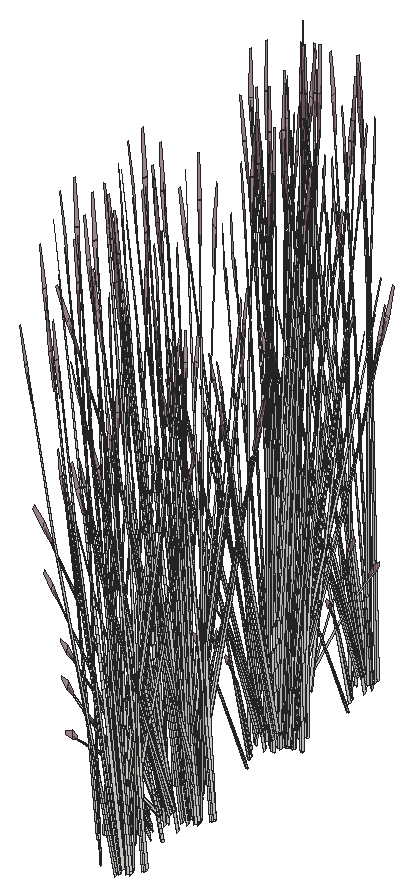
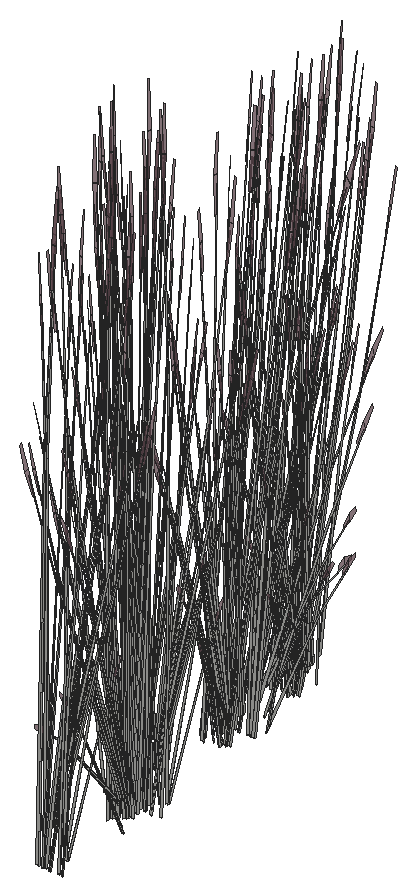
# SketchUp Ruby script. Lengths in inches.
U = 1.inch
M = Sketchup.active_model
def pt(a) = Geom::Point3d.new(a.map { |v| v * U })
def face(e, loops, mat)
  f = e.add_face(loops[0].map { |a| pt(a) })
  loops[1..].each { |l| e.add_face(l.map { |a| pt(a) }).erase! }
  f.material = f.back_material = mat if mat
  f
end
# faces: each face lists its corners as indices into pts; further lists are holes
def faces(e, pts, list, mat = nil) = list.each { |f| face(e, (f[0].is_a?(Array) ? f : [f]).map { |l| l.map { |i| pts[i] } }, mat) }
# xy, xz, yz: faces in a plane at the given z, y or x. An outline is a flat list of corners, or four numbers for a rectangle; further outlines are holes
def ring(l) = l.size == 4 ? [[l[0], l[1]], [l[2], l[1]], [l[2], l[3]], [l[0], l[3]]] : l.each_slice(2).to_a
def flat(e, list, mat, &to3) = list.each { |f| face(e, (f[0].is_a?(Array) ? f : [f]).map { |l| ring(l).map { |u, v| to3.(u, v) } }, mat) }
def xy(e, z, list, mat = nil) = flat(e, list, mat) { |x, y| [x, y, z] }
def xz(e, y, list, mat = nil) = flat(e, list, mat) { |x, z| [x, y, z] }
def yz(e, x, list, mat = nil) = flat(e, list, mat) { |y, z| [x, y, z] }
def lines(e, pts, list) = list.each { |a, b| e.add_line(pt(pts[a]), pt(pts[b])) }
# prism: a flat outline (further loops are holes) pulled along v
def prism(e, loops, v, mat = nil)
  f = face(e, loops, mat); d = Geom::Vector3d.new(v.map { |x| x * U })
  f.pushpull(f.normal.samedirection?(d) ? d.length : -d.length)
end
def box(e, o, s, mat = nil) = prism(e, [[o, [o[0] + s[0], o[1], o[2]], [o[0] + s[0], o[1] + s[1], o[2]], [o[0], o[1] + s[1], o[2]]]], [0, 0, s[2]], mat)
def at(x, y, z, deg = 0) = Geom::Transformation.translation(pt([x, y, z])) * Geom::Transformation.rotation(ORIGIN, Z_AXIS, deg.degrees)
def axes(o, x, y, z) = Geom::Transformation.new([*x, 0, *y, 0, *z, 0, *pt(o).to_a, 1])
def part(name) = M.definitions.add(name)
# library, detail: a bought-in or finely detailed component or shape, given as its bounding box
def library(name, o, s) = part(name).tap { |d| box(d.entities, o, s) }
def detail(e, o, s) = box(e.add_group.entities, o, s)
def put(e, d, t, mat = nil) = e.add_instance(d, t).tap { |i| i.material = mat if mat }
def group(e, t, mat = nil) = e.add_group.tap { |g| g.transformation = t; g.material = mat if mat }.entities
root = M.entities
M.materials.add("LightPink_Translucent").color = [144, 107, 117]
M.materials["LightPink_Translucent"].alpha = 0.75
c1 = part("blade")
p = [[2.15,0.21,22],[0,0.17,0],[0.09,0.45,0],[2.18,0.31,22],[2.29,0.31,22],[0.38,0.45,0],
  [2.48,0.24,33],[2.49,0.24,33],[2.48,0.22,33]]
faces(c1.entities,p,[[0,1,2,3],[4,5,2,3],[6,3,4,7],[8,0,3,6]])
c2 = part("seeds")
p = [[0.3,-0.1,1.38],[-0.01,-0.03,1.59],[-0.01,-0.03,0.03],[0.14,-0.07,-0.07],[0.29,-0.03,3],[0.15,0.01,3.11]]
faces(c2.entities,p,[[0,1,2,3],[1,0,4,5]],"LightPink_Translucent")
c3 = part("blade with seeds")
put(c3.entities,c1,at(0,0,0))
put(c3.entities,c2,axes([2.4,0.25,30.99],[1.5799,-0.05474,1.17369],[-0.12525,1.92788,0.29478],[-0.07173,-0.02425,1.56792]))
put(root,c3,axes([405.85,331.17,-9.69],[0,0.54355,0.46235],[-0.57217,0,0],[0,-0.1238,1.46668]))
put(root,c3,axes([407.2,331.61,-9.94],[-0.30722,-0.45622,-0.41661],[0.46535,-0.32126,0.2005],[-0.09942,-0.05645,1.33761]))
put(root,c3,axes([406.93,331.78,-10.08],[-0.53199,-0.08911,-0.58063],[0.11226,-0.54969,-0.15239],[-0.15876,-0.06661,1.28164]))
put(root,c3,axes([406.36,332.62,-10.11],[-0.12013,-0.47362,-0.28847],[0.47712,-0.13449,0.28847],[-0.09619,-0.05462,1.29413]))
put(root,c3,axes([406.23,332.82,-10.12],[-0.47863,-0.27177,-0.46235],[0.28609,-0.48733,0],[-0.10901,-0.0619,1.46668]))
put(root,c3,axes([407.53,331.86,-9.52],[-0.51635,0.36087,-0.27094],[-0.34336,-0.5099,-0.46562],[-0.1274,-0.05178,1.4872]))
put(root,c3,axes([407.48,332.02,-9.5625],[-0.09866,0.48509,0.13483],[-0.48202,-0.0842,-0.38503],[-0.08772,-0.04981,1.18024]))
put(root,c3,axes([405.61,330.76,-7.3],[0.42502,0.15163,0.32977],[-0.12396,0.44238,-0.42575],[-0.17112,0.04056,0.81462]))
put(root,c3,axes([408.11,332.03,-9.7],[-0.49938,-0.43748,-0.23459],[0.42021,-0.49126,0.51337],[-0.13447,0.05118,1.56642]))
put(root,c3,axes([406.8,332.87,-9.69],[0.47863,0.27177,0.46235],[-0.28609,0.48733,0],[-0.10901,-0.0619,1.46668]))
put(root,c3,axes([406.52,333.15,-9.79],[-0.31974,0.54466,0],[-0.53494,-0.30375,-0.48057],[-0.12184,-0.06918,1.52448]))
put(root,c3,axes([407.86,331.93,-9.94],[-0.55535,0.03355,-0.41661],[-0.05022,-0.55698,0.2005],[-0.09942,0.05645,1.33761]))
put(root,c3,axes([405.78,337.88,-8.39],[0.1169,0.17452,1.59586],[-0.54019,0.14692,0.12904],[-0.12209,-0.27397,0.68222]))
put(root,c3,axes([408.47,333.23,-9.96],[-0.31576,-0.54657,-0.04789],[0.53494,-0.30375,0.48057],[-0.13182,0.05204,1.52373]))
put(root,c3,axes([406.67,336.73,-7.61],[-0.07822,-0.07621,1.62908],[-0.52201,0.04832,-0.25764],[-0.08331,-0.18228,0.13065]))
put(root,c3,axes([407.21,338.01,-7.36],[-0.24409,-0.44196,-0.66157],[0.50245,-0.2463,0.07984],[-0.05708,-0.21354,0.93586]))
put(root,c3,axes([405.63,337.42,-9.59],[-0.03097,0.17781,1.33163],[-0.45273,0.14885,-0.28638],[-0.10583,-0.22982,0.56934]))
put(root,c3,axes([408.33,333.16,-10.11],[-0.47712,-0.13449,-0.28847],[0.12013,-0.47362,0.28847],[-0.09619,0.05462,1.29413]))
put(root,c3,axes([405.68,331.82,-7.3],[0.44516,-0.07768,0.32977],[0.11755,0.44407,-0.42575],[-0.12757,0.11927,0.81462]))
put(root,c3,axes([407.03,337.93,-7.64],[-0.50273,-0.13626,-0.47583],[0.17232,-0.46717,-0.36857],[-0.0461,-0.18809,0.91046]))
put(root,c3,axes([406.13,336.48,-7.62],[-0.00954,0.06515,1.65179],[-0.47055,0.23645,-0.15608],[-0.13847,-0.12087,0.29231]))
put(root,c3,axes([404.67,333.08,-6.74],[0.45129,0.14509,-0.06041],[-0.13882,0.44656,-0.27392],[-0.07381,0.0678,0.90349]))
put(root,c3,axes([407.87,332.26,-10.08],[-0.34446,0.40855,-0.58063],[-0.42791,-0.37046,-0.15239],[-0.13803,0.10191,1.28164]))
put(root,c3,axes([406.03,337.63,-7.26],[0.56969,-0.13971,0.50064],[0.09887,0.54803,0.4128],[-0.13398,-0.16152,1.03595]))
put(root,c3,axes([407.46,337.9,-7.3125],[-0.50045,0.25306,-0.11324],[-0.24593,-0.44915,-0.62851],[-0.06603,-0.18927,0.95501]))
put(root,c3,axes([408.44,333.37,-10.12],[-0.47863,0.27177,-0.46235],[-0.28609,-0.48733,0],[-0.10901,0.0619,1.46668]))
put(root,c3,axes([405.47,337.14,-9.42],[0.26677,0.18918,1.06958],[-0.38851,0.11372,0.78586],[-0.08313,-0.14539,0.23558]))
put(root,c3,axes([405.96,337.79,-7.78],[-0.07899,-0.43781,-0.32977],[0.45153,-0.11561,0.42575],[-0.12128,-0.12546,0.81462]))
put(root,c3,axes([405.45,331.78,-7.3125],[0.47307,0.29971,-0.11324],[-0.27254,0.43404,-0.62851],[-0.13365,0.15087,0.95501]))
put(root,c3,axes([405.6875,332.14,-7.64],[0.13138,0.49631,-0.47583],[-0.49754,0.08682,-0.36857],[-0.14258,0.13331,0.91046]))
put(root,c3,axes([406.16,337.75,-7.6],[0.23243,-0.34529,0.05988],[0.331,0.20103,0.47138],[-0.10701,-0.1107,0.71878]))
put(root,c3,axes([405.26,337.71,-10.61],[-0.04954,0.0716,1.6421],[-0.50062,0.15438,-0.25086],[-0.12094,-0.14044,0.2797]))
put(root,c3,axes([406.28,332.71,-7.3],[0.34603,-0.28618,0.32977],[0.32756,0.32677,-0.42575],[-0.04984,0.16603,0.81462]))
put(root,c3,axes([406.09,339.67,-10.05],[-0.21003,-0.55738,-0.65031],[0.60499,-0.20074,-0.17068],[-0.02321,-0.18874,1.43544]))
put(root,c3,axes([408.6,331.13,-9.35],[-0.01397,-0.51177,1.31553],[0.63227,0.13266,0.557],[-0.14954,0.28003,1.24175]))
put(root,c3,axes([405.97,332.97,-7.6],[-0.42027,-0.02533,0.05988],[0.01152,-0.38243,0.47138],[-0.04398,0.14649,0.71878]))
put(root,c3,axes([406.1,333,-7.59],[-0.36417,-0.37086,0.447],[0.38674,-0.31985,0.36857],[-0.06718,0.174,0.92496]))
put(root,c3,axes([406.71,337.42,-10.02],[-0.35341,0.31182,-0.03625],[-0.32382,-0.34152,-0.16435],[-0.0228,-0.09677,0.54209]))
put(root,c3,axes([405.99,332.0625,-8.39],[0.09522,-0.18683,1.59586],[0.39947,0.38663,0.12904],[-0.18021,0.24097,0.68222]))
put(root,c3,axes([407.16,341.11,-8.9],[0.44194,0.21918,1.40854],[-0.43295,0.47219,0.557],[-0.19393,-0.27986,1.18082]))
put(root,c3,axes([406.1,333.11,-7.78],[-0.34603,0.28618,-0.32977],[-0.32756,-0.32677,0.42575],[-0.04984,0.16603,0.81462]))
put(root,c3,axes([404.91,333.03,-7.61],[-0.01271,0.10756,1.62908],[0.36076,0.37419,-0.25764],[-0.09444,0.17695,0.13065]))
put(root,c3,axes([406.0625,332.79,-6.97],[0.56206,0.02693,-0.12569],[-0.01536,0.50991,-0.69765],[-0.03904,0.19638,1.06006]))
put(root,c3,axes([406.23,338.15,-7.3],[0.07899,0.43781,0.32977],[-0.45153,0.11561,-0.42575],[-0.12128,-0.12546,0.81462]))
put(root,c3,axes([404.85,339.6,-10.12],[0,-0.54355,-0.46235],[0.57217,0,0],[0,-0.1238,1.46668]))
put(root,c3,axes([406.32,334.23,-9.42],[-0.01324,-0.32319,1.06958],[0.33072,0.23052,0.78586],[-0.06504,0.15405,0.23558]))
put(root,c3,axes([406.45,332.98,-7.34],[0.3661,0.36521,-0.52818],[-0.38674,0.31985,-0.40911],[-0.0557,0.18556,1.01061]))
put(root,c3,axes([406.05,333.53,-9.37],[0.46459,-0.09625,0.0606],[0.10681,0.38778,-0.80367],[-0.02945,0.1963,0.72038]))
put(root,c3,axes([405.09,339.61,-10.11],[0.35699,-0.33913,-0.28847],[0.35699,0.33913,0.28847],[0,-0.10923,1.29413]))
put(root,c3,axes([404.95,337.98,-10.02],[-0.14753,0.44383,-0.03625],[-0.45406,-0.13653,-0.16435],[-0.06894,-0.07259,0.54209]))
put(root,c3,axes([406.34,340.23,-9.52],[-0.57594,-0.25935,-0.27094],[0.27732,-0.5474,-0.46562],[-0.0181,-0.1344,1.4872]))
put(root,c3,axes([404.71,340.01,-9.79],[-0.63949,0,0],[0,-0.60749,-0.48057],[0,-0.13836,1.52448]))
put(root,c3,axes([406.33,332.8125,-7.03],[-0.01331,0.50278,-0.73435],[-0.56035,-0.03377,0.08862],[-0.05914,0.213,1.03881]))
put(root,c3,axes([404.87,334.13,-7.62],[0.05802,-0.03282,1.65179],[0.47954,0.21828,-0.15608],[-0.01127,0.18175,0.29231]))
put(root,c3,axes([405.9375,333.9375,-9.59],[0.16138,-0.08575,1.33163],[0.39845,0.25854,-0.28638],[-0.1186,0.22371,0.56934]))
put(root,c3,axes([405.2,339.85,-9.83],[-0.47569,0.45698,0.2864],[-0.47598,-0.45217,-0.33981],[-0.01661,-0.12977,1.53541]))
put(root,c3,axes([406.49,340.8,-9.73],[0.13555,-0.64407,-0.21817],[0.64269,0.11227,0.47743],[-0.1123,-0.08895,1.45677]))
put(root,c3,axes([406.15,333.52,-8.87],[0.01124,-0.2806,1.43727],[0.50537,0.14821,0.19862],[-0.04379,0.29905,0.67868]))
put(root,c3,axes([405.09,340.1,-9.69],[0,0.54355,0.46235],[-0.57217,0,0],[0,-0.1238,1.46668]))
put(root,c3,axes([406.44,340.54,-9.94],[-0.30722,-0.45622,-0.41661],[0.46535,-0.32126,0.2005],[-0.09942,-0.05645,1.33761]))
put(root,c3,axes([406.4,340.375,-9.47],[-0.24813,0.48978,0.41661],[-0.51557,-0.23571,-0.2005],[0,-0.1129,1.33761]))
put(root,c3,axes([406.5625,340.49,-9.8],[0.64638,0.11452,0.42607],[-0.13155,0.64678,0.16719],[-0.09446,-0.06245,1.47927]))
put(root,c3,axes([405.6,341.55,-10.11],[-0.12013,-0.47362,-0.28847],[0.47712,-0.13449,0.28847],[-0.09619,-0.05462,1.29413]))
put(root,c3,axes([406.22,341.52,-9.7],[0.54955,-0.14427,0.16428],[0.1357,0.53689,0.32672],[-0.04901,-0.07823,1.49371]))
put(root,c3,axes([405.47,341.76,-10.12],[-0.47863,-0.27177,-0.46235],[0.28609,-0.48733,0],[-0.10901,-0.0619,1.46668]))
put(root,c3,axes([406.77,340.8,-9.52],[-0.51635,0.36087,-0.27094],[-0.34336,-0.5099,-0.46562],[-0.1274,-0.05178,1.4872]))
put(root,c3,axes([406.72,340.95,-9.5625],[-0.09866,0.48509,0.13483],[-0.48202,-0.0842,-0.38503],[-0.08772,-0.04981,1.18024]))
put(root,c3,axes([407.35,340.96,-9.7],[-0.49938,-0.43748,-0.23459],[0.42021,-0.49126,0.51337],[-0.13447,0.05118,1.56642]))
put(root,c3,axes([406.04,341.8,-9.69],[0.47863,0.27177,0.46235],[-0.28609,0.48733,0],[-0.10901,-0.0619,1.46668]))
put(root,c3,axes([405.76,342.08,-9.79],[-0.31974,0.54466,0],[-0.53494,-0.30375,-0.48057],[-0.12184,-0.06918,1.52448]))
put(root,c3,axes([407.1,340.87,-9.94],[-0.55535,0.03355,-0.41661],[-0.05022,-0.55698,0.2005],[-0.09942,0.05645,1.33761]))
put(root,c3,axes([407.71,342.16,-9.96],[-0.31576,-0.54657,-0.04789],[0.53494,-0.30375,0.48057],[-0.13182,0.05204,1.52373]))
put(root,c3,axes([407.57,342.09,-10.11],[-0.47712,-0.13449,-0.28847],[0.12013,-0.47362,0.28847],[-0.09619,0.05462,1.29413]))
put(root,c3,axes([404.92,340.76,-7.3],[0.44516,-0.07768,0.32977],[0.11755,0.44407,-0.42575],[-0.12757,0.11927,0.81462]))
put(root,c3,axes([407.49,340.72,-9.52],[0.05959,0.62022,-0.27094],[-0.62068,0.0375,-0.46562],[-0.1093,0.08261,1.4872]))
put(root,c3,axes([403.91,342.02,-6.74],[0.45129,0.14509,-0.06041],[-0.13882,0.44656,-0.27392],[-0.07381,0.0678,0.90349]))
put(root,c3,axes([407.11,341.19,-10.08],[-0.34446,0.40855,-0.58063],[-0.42791,-0.37046,-0.15239],[-0.13803,0.10191,1.28164]))
put(root,c3,axes([407.68,342.31,-10.12],[-0.47863,0.27177,-0.46235],[-0.28609,-0.48733,0],[-0.10901,0.0619,1.46668]))
put(root,c3,axes([404.69,340.72,-7.3125],[0.47307,0.29971,-0.11324],[-0.27254,0.43404,-0.62851],[-0.13365,0.15087,0.95501]))
put(root,c3,axes([405.52,341.64,-7.3],[0.34603,-0.28618,0.32977],[0.32756,0.32677,-0.42575],[-0.04984,0.16603,0.81462]))
put(root,c3,axes([407.84,340.06,-9.35],[-0.01397,-0.51177,1.31553],[0.63227,0.13266,0.557],[-0.14954,0.28003,1.24175]))
put(root,c3,axes([405.21,341.9,-7.6],[-0.42027,-0.02533,0.05988],[0.01152,-0.38243,0.47138],[-0.04398,0.14649,0.71878]))
put(root,c3,axes([405.34,341.9375,-7.59],[-0.36417,-0.37086,0.447],[0.38674,-0.31985,0.36857],[-0.06718,0.174,0.92496]))
put(root,c3,axes([405.34,342.05,-7.78],[-0.34603,0.28618,-0.32977],[-0.32756,-0.32677,0.42575],[-0.04984,0.16603,0.81462]))
put(root,c3,axes([405.3,341.72,-6.97],[0.56206,0.02693,-0.12569],[-0.01536,0.50991,-0.69765],[-0.03904,0.19638,1.06006]))
put(root,c3,axes([405.5625,343.16,-9.42],[-0.01324,-0.32319,1.06958],[0.33072,0.23052,0.78586],[-0.06504,0.15405,0.23558]))
put(root,c3,axes([405.6875,341.91,-7.34],[0.3661,0.36521,-0.52818],[-0.38674,0.31985,-0.40911],[-0.0557,0.18556,1.01061]))
put(root,c3,axes([405.29,342.46,-9.37],[0.46459,-0.09625,0.0606],[0.10681,0.38778,-0.80367],[-0.02945,0.1963,0.72038]))
put(root,c3,axes([405.57,341.74,-7.03],[-0.01331,0.50278,-0.73435],[-0.56035,-0.03377,0.08862],[-0.05914,0.213,1.03881]))
put(root,c3,axes([404.11,343.07,-7.62],[0.05802,-0.03282,1.65179],[0.47954,0.21828,-0.15608],[-0.01127,0.18175,0.29231]))
put(root,c3,axes([406.1,341.39,-8.39],[-0.01252,-0.20862,1.59586],[0.54251,0.1384,0.12904],[-0.03356,0.2973,0.68222]))
put(root,c3,axes([405.18,342.87,-9.59],[0.16138,-0.08575,1.33163],[0.39845,0.25854,-0.28638],[-0.1186,0.22371,0.56934]))
put(root,c3,axes([404.54,351.54,-7.36],[-0.24409,-0.44196,-0.66157],[0.50245,-0.2463,0.07984],[-0.05708,-0.21354,0.93586]))
put(root,c3,axes([404.12,350.5625,-10.61],[-0.08578,0.01958,1.6421],[-0.47437,-0.22044,-0.25086],[0.00796,-0.18387,0.2797]))
put(root,c3,axes([405.39,342.45,-8.87],[0.01124,-0.2806,1.43727],[0.50537,0.14821,0.19862],[-0.04379,0.29905,0.67868]))
put(root,c3,axes([404.58,351.17,-7.78],[0.15418,-0.41799,-0.32977],[0.44981,0.12192,0.42575],[-0.04124,-0.16829,0.81462]))
put(root,c3,axes([406.22,350.8,-7.62],[-0.05194,0.04152,1.65179],[-0.50886,-0.14007,-0.15608],[-0.01842,-0.18118,0.29231]))
put(root,c3,axes([404.35,351.46,-7.64],[-0.50273,-0.13626,-0.47583],[0.17232,-0.46717,-0.36857],[-0.0461,-0.18809,0.91046]))
put(root,c3,axes([404.67,350.29,-9.42],[0.06561,0.31695,1.06958],[-0.36394,-0.17555,0.78586],[0.03916,-0.16229,0.23558]))
put(root,c3,axes([405.44,351.81,-7.64],[-0.3661,-0.36521,-0.47583],[0.38674,-0.31985,-0.36857],[0.0557,-0.18556,0.91046]))
put(root,c3,axes([404.64,351.27,-7.59],[0.50393,0.1421,0.447],[-0.17232,0.46717,0.36857],[-0.03028,-0.18372,0.92496]))
put(root,c3,axes([404.78,351.43,-7.3125],[-0.50045,0.25306,-0.11324],[-0.24593,-0.44915,-0.62851],[-0.06603,-0.18927,0.95501]))
put(root,c3,axes([405.82,352,-7.3125],[-0.56206,-0.02693,-0.11324],[0.01536,-0.50991,-0.62851],[0.03904,-0.19638,0.95501]))
put(root,c3,axes([404.77,351.23,-7.6],[0.37684,-0.18473,0.05988],[0.18445,0.33686,0.47138],[-0.03639,-0.14849,0.71878]))
put(root,c3,axes([403.41,353.21,-10.05],[-0.21003,-0.55738,-0.65031],[0.60499,-0.20074,-0.17068],[-0.02321,-0.18874,1.43544]))
put(root,c3,axes([404.63,351.61,-7.3],[-0.15418,0.41799,0.32977],[-0.44981,-0.12192,-0.42575],[-0.04124,-0.16829,0.81462]))
put(root,c3,axes([405.6,352.08,-7.3],[-0.34603,0.28618,0.32977],[-0.32756,-0.32677,-0.42575],[0.04984,-0.16603,0.81462]))
put(root,c3,axes([403.33,351.6,-9.79],[-0.31974,-0.54466,0],[0.53494,-0.30375,-0.48057],[0.12184,-0.06918,1.52448]))
put(root,c3,axes([404.03,350.95,-10.02],[-0.35341,0.31182,-0.03625],[-0.32382,-0.34152,-0.16435],[-0.0228,-0.09677,0.54209]))
put(root,c3,axes([403.73,353.35,-9.94],[0.24813,-0.48978,-0.41661],[0.51557,0.23571,0.2005],[0,-0.1129,1.33761]))
put(root,c3,axes([403.96,353.11,-9.52],[-0.05959,-0.62022,-0.27094],[0.62068,-0.0375,-0.46562],[0.1093,-0.08261,1.4872]))
put(root,c3,axes([402.42,353.14,-10.11],[0.35699,-0.33913,-0.28847],[0.35699,0.33913,0.28847],[0,-0.10923,1.29413]))
put(root,c3,axes([404.04,353.59,-9.73],[0.57623,0.26344,0.22409],[-0.27732,0.5474,0.46562],[0,-0.12618,1.49497]))
put(root,c3,axes([403.85,353.23,-9.47],[-0.55535,0.03355,0.41661],[-0.05022,-0.55698,-0.2005],[0.09942,-0.05645,1.33761]))
put(root,c3,axes([403.83,353.43,-9.8],[0.22235,0.6078,0.42607],[-0.63531,0.21135,0.16719],[0.00776,-0.11168,1.47927]))
put(root,c3,axes([403.72,353.9,-9.47],[-0.24813,0.48978,0.41661],[-0.51557,-0.23571,-0.2005],[0,-0.1129,1.33761]))
put(root,c3,axes([404.63,353.48,-9.95],[0,-0.62892,0],[0.63949,0,0],[0,0,1.6711]))
put(root,c3,axes([404.33,353.08,-9.8],[-0.42403,0.49328,0.42607],[-0.50377,-0.43543,0.16719],[0.10223,-0.04923,1.47927]))
put(root,c3,axes([404.79,353.96,-9.86],[-0.47569,-0.46784,-0.05709],[0.47598,-0.46812,0],[-0.01661,-0.01634,1.63492]))
put(root,c3,axes([403.59,352.27,-9.7],[-0.14774,0.54019,0.16428],[-0.54062,-0.15287,0.32672],[0.09339,-0.00263,1.49371]))
put(root,c3,axes([403.89,354.02,-9.8],[0.64638,0.11452,0.42607],[-0.13155,0.64678,0.16719],[-0.09446,-0.06245,1.47927]))
put(root,c3,axes([404.51,353,-9.47],[-0.30722,-0.45622,0.41661],[0.46535,-0.32126,-0.2005],[0.09942,0.05645,1.33761]))
put(root,c3,axes([403.54,355.05,-9.7],[0.54955,-0.14427,0.16428],[0.1357,0.53689,0.32672],[-0.04901,-0.07823,1.49371]))
put(root,c3,axes([405.06,353.62,-9.95],[0.57217,0,0],[0,0.56272,0],[0,0,1.66132]))
put(root,c3,axes([405.23,352.3,-9.7],[-0.54955,0.14427,0.16428],[-0.1357,-0.53689,0.32672],[0.04901,0.07823,1.49371]))
put(root,c3,axes([404.88,353.33,-9.78],[-0.64638,-0.11452,0.45814],[0.13155,-0.64678,0.17978],[0.09446,0.06245,1.59061]))
put(root,c3,axes([404.36,354.93,-9.95],[-0.16686,-0.46861,0],[0.47648,-0.16411,0],[0,0,1.4375]))
put(root,c3,axes([405.17,355.08,-9.7],[0.14774,-0.54019,0.16428],[0.54062,0.15287,0.32672],[-0.09339,0.00263,1.49371]))
put(root,c3,axes([405.05,353.86,-9.9375],[0.35699,0.35109,0],[-0.35699,0.35109,0],[0,0,1.57621]))
put(root,c3,axes([406.02,353.71,-9.7],[-0.40181,-0.39593,0.16428],[0.40492,-0.38402,0.32672],[-0.04438,0.08086,1.49371]))
put(root,c3,axes([404.25,355.14,-9.95],[-0.51557,-0.24403,0],[0.24813,-0.50705,0],[0,0,1.51513]))
put(root,c3,axes([405.05,353.45,-9.47],[0.24813,-0.48978,0.41661],[0.51557,0.23571,-0.2005],[0,0.1129,1.33761]))
put(root,c3,axes([404.95,353.73,-9.87],[0,0.62861,-0.05249],[-0.63949,0,0],[0,0.01975,1.67027]))
put(root,c3,axes([404.92,354.13,-9.47],[0.55535,-0.03355,0.41661],[0.05022,0.55698,-0.2005],[-0.09942,0.05645,1.33761]))
put(root,c3,axes([405.26,353.56,-9.5625],[0.47648,-0.15851,0.13483],[0.16686,0.45265,-0.38503],[0,0.09962,1.18024]))
put(root,c3,axes([404.83,355.15,-9.95],[0.51557,0.24403,0],[-0.24813,0.50705,0],[0,0,1.62917]))
put(root,c3,axes([404.93,354.37,-9.5625],[0.37783,0.32657,0.13483],[-0.31516,0.36844,-0.38503],[-0.08772,0.04981,1.18024]))
put(root,c3,axes([405.33,355.375,-9.69],[0.47863,-0.27177,0.46235],[0.28609,0.48733,0],[-0.10901,0.0619,1.46668]))
put(root,c3,axes([404.65,354.94,-9.87],[0.22235,0.62444,-0.05599],[-0.63531,0.21881,0],[0.00776,0.02181,1.60327]))
put(root,c3,axes([406.48,354.125,-9.95],[-0.63917,-0.00435,-0.04634],[0,-0.60749,0.46507],[-0.02009,0.13829,1.47457]))
put(root,c3,axes([405.1,353.6,-9.52],[0.57594,0.25935,-0.27094],[-0.27732,0.5474,-0.46562],[0.0181,0.1344,1.4872]))
put(root,c3,axes([406.35,354.21,-10.11],[-0.35699,0.33913,-0.28847],[-0.35699,-0.33913,0.28847],[0,0.10923,1.29413]))
put(root,c3,axes([404.8125,354.25,-9.52],[0.05959,0.62022,-0.27094],[-0.62068,0.0375,-0.46562],[-0.1093,0.08261,1.4872]))
put(root,c3,axes([405.04,354,-9.94],[-0.24813,0.48978,-0.41661],[-0.51557,-0.23571,0.2005],[0,0.1129,1.33761]))
put(root,c3,axes([405.05,355.41,-9.83],[0.64025,0.17667,0.2864],[-0.16018,0.63149,-0.33981],[-0.10597,0.07904,1.53541]))
put(root,c3,axes([405.44,355.75,-9.79],[0.31974,0.54466,0],[-0.53494,0.30375,-0.48057],[-0.12184,0.06918,1.52448]))
put(root,c3,axes([405.33,354.15,-10.05],[0.18752,0.49766,-0.6445],[-0.54017,0.17923,-0.16915],[0.02073,0.16852,1.42262]))
put(root,c3,axes([403.82,355.64,-7.3],[0.15418,-0.41799,0.32977],[0.44981,0.12192,-0.42575],[0.04124,0.16829,0.81462]))
put(root,c3,axes([405.05,362.75,-7.36],[-0.24409,-0.44196,-0.66157],[0.50245,-0.2463,0.07984],[-0.05708,-0.21354,0.93586]))
put(root,c3,axes([404.63,361.77,-10.61],[-0.08578,0.01958,1.6421],[-0.47437,-0.22044,-0.25086],[0.00796,-0.18387,0.2797]))
put(root,c3,axes([404.42,357.13,-6.74],[0.35341,-0.31182,-0.06041],[0.32382,0.34152,-0.27392],[0.0228,0.09677,0.90349]))
put(root,c3,axes([405.1,362.375,-7.78],[0.15418,-0.41799,-0.32977],[0.44981,0.12192,0.42575],[-0.04124,-0.16829,0.81462]))
put(root,c3,axes([403.68,356.02,-7.6],[-0.37684,0.18473,0.05988],[-0.18445,-0.33686,0.47138],[0.03639,0.14849,0.71878]))
put(root,c3,axes([404.87,362.66,-7.64],[-0.50273,-0.13626,-0.47583],[0.17232,-0.46717,-0.36857],[-0.0461,-0.18809,0.91046]))
put(root,c3,axes([405.18,361.49,-9.42],[0.06561,0.31695,1.06958],[-0.36394,-0.17555,0.78586],[0.03916,-0.16229,0.23558]))
put(root,c3,axes([403.67,355.82,-7.3125],[0.50045,-0.25306,-0.11324],[0.24593,0.44915,-0.62851],[0.06603,0.18927,0.95501]))
put(root,c3,axes([403.8125,355.99,-7.28],[-0.50393,-0.1421,0.49617],[0.17232,-0.46717,0.40911],[0.03028,0.18372,1.0267]))
put(root,c3,axes([403.76,355.92,-10.61],[0.08277,-0.02958,1.6421],[0.49786,0.16279,-0.25086],[0.01456,0.18348,0.2797]))
put(root,c3,axes([405.16,362.47,-7.59],[0.50393,0.1421,0.447],[-0.17232,0.46717,0.36857],[-0.03028,-0.18372,0.92496]))
put(root,c3,axes([405.3,362.64,-7.3125],[-0.50045,0.25306,-0.11324],[-0.24593,-0.44915,-0.62851],[-0.06603,-0.18927,0.95501]))
put(root,c3,axes([404.1,355.8,-7.64],[0.50273,0.13626,-0.47583],[-0.17232,0.46717,-0.36857],[0.0461,0.18809,0.91046]))
put(root,c3,axes([405.29,362.44,-7.6],[0.37684,-0.18473,0.05988],[0.18445,0.33686,0.47138],[-0.03639,-0.14849,0.71878]))
put(root,c3,axes([403.87,356.08,-7.78],[-0.15418,0.41799,-0.32977],[-0.44981,-0.12192,0.42575],[0.04124,0.16829,0.81462]))
put(root,c3,axes([403.43,354.92,-8.39],[-0.01252,-0.20862,1.59586],[0.54251,0.1384,0.12904],[-0.03356,0.2973,0.68222]))
put(root,c3,axes([403.92,364.41,-10.05],[-0.21003,-0.55738,-0.65031],[0.60499,-0.20074,-0.17068],[-0.02321,-0.18874,1.43544]))
put(root,c3,axes([403.91,355.71,-7.36],[0.24409,0.44196,-0.66157],[-0.50245,0.2463,0.07984],[0.05708,0.21354,0.93586]))
put(root,c3,axes([405.15,362.8125,-7.3],[-0.15418,0.41799,0.32977],[-0.44981,-0.12192,-0.42575],[-0.04124,-0.16829,0.81462]))
put(root,c3,axes([403.55,356.82,-7.61],[0.06483,0.08753,1.62908],[0.52315,0.03439,-0.25764],[0.05261,0.19303,0.13065]))
put(root,c3,axes([403.84,362.81,-9.79],[-0.31974,-0.54466,0],[0.53494,-0.30375,-0.48057],[0.12184,-0.06918,1.52448]))
put(root,c3,axes([404.54,362.15,-10.02],[-0.35341,0.31182,-0.03625],[-0.32382,-0.34152,-0.16435],[-0.0228,-0.09677,0.54209]))
put(root,c3,axes([402.6875,364.33,-10.12],[0,-0.54355,-0.46235],[0.57217,0,0],[0,-0.1238,1.46668]))
put(root,c3,axes([404.24,364.55,-9.94],[0.24813,-0.48978,-0.41661],[0.51557,0.23571,0.2005],[0,-0.1129,1.33761]))
put(root,c3,axes([402.93,364.34,-10.11],[0.35699,-0.33913,-0.28847],[0.35699,0.33913,0.28847],[0,-0.10923,1.29413]))
put(root,c3,axes([404.18,364.96,-9.52],[-0.57594,-0.25935,-0.27094],[0.27732,-0.5474,-0.46562],[-0.0181,-0.1344,1.4872]))
put(root,c3,axes([404.55,364.8,-9.73],[0.57623,0.26344,0.22409],[-0.27732,0.5474,0.46562],[0,-0.12618,1.49497]))
put(root,c3,axes([404.37,364.43,-9.47],[-0.55535,0.03355,0.41661],[-0.05022,-0.55698,-0.2005],[0.09942,-0.05645,1.33761]))
put(root,c3,axes([402.93,364.84,-9.69],[0,0.54355,0.46235],[-0.57217,0,0],[0,-0.1238,1.46668]))
put(root,c3,axes([404.35,364.63,-9.8],[0.22235,0.6078,0.42607],[-0.63531,0.21135,0.16719],[0.00776,-0.11168,1.47927]))
put(root,c3,axes([404.23,365.11,-9.47],[-0.24813,0.48978,0.41661],[-0.51557,-0.23571,-0.2005],[0,-0.1129,1.33761]))
